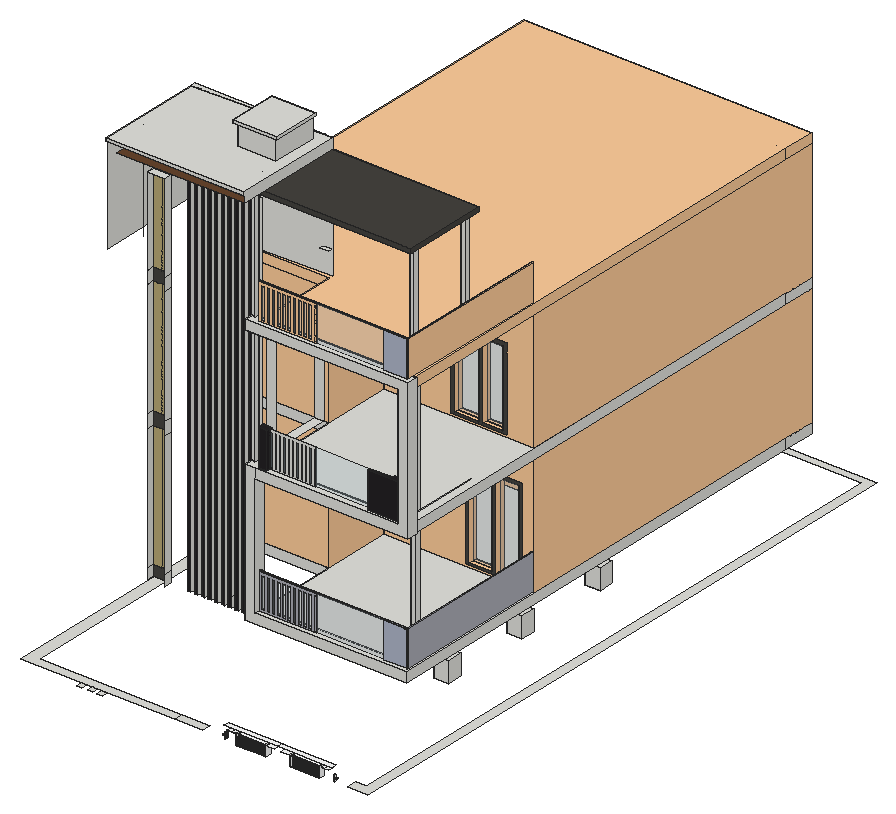
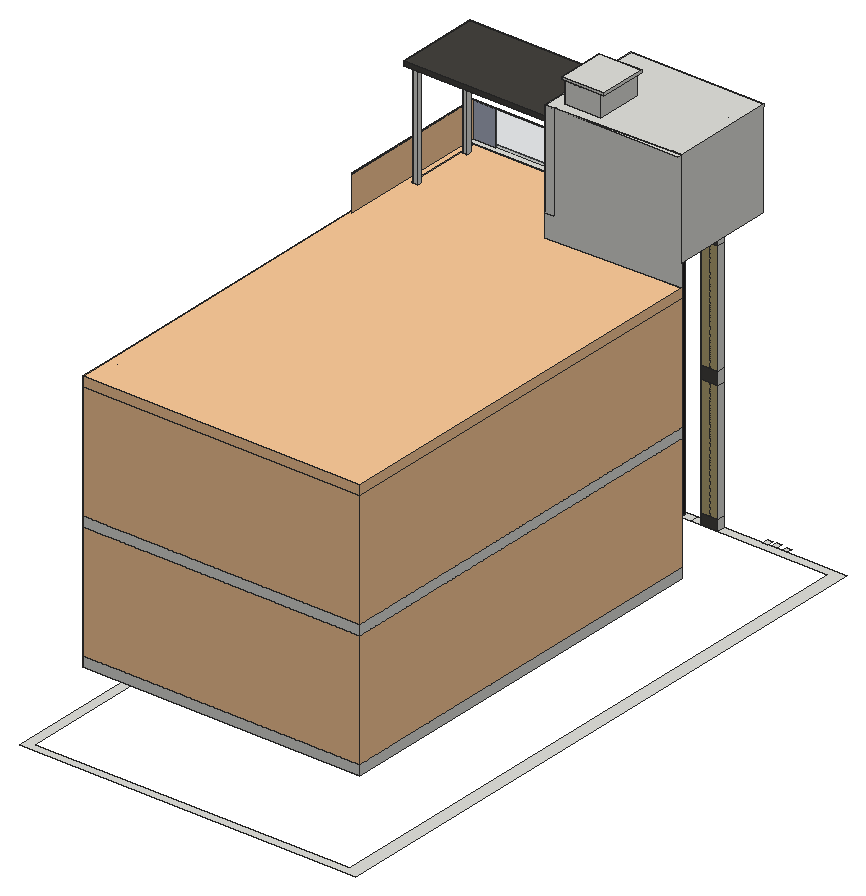
# SketchUp Ruby script. Lengths in inches.
U = 1.inch
M = Sketchup.active_model
def pt(a) = Geom::Point3d.new(a.map { |v| v * U })
def face(e, loops, mat)
  f = e.add_face(loops[0].map { |a| pt(a) })
  loops[1..].each { |l| e.add_face(l.map { |a| pt(a) }).erase! }
  f.material = f.back_material = mat if mat
  f
end
# faces: each face lists its corners as indices into pts; further lists are holes
def faces(e, pts, list, mat = nil) = list.each { |f| face(e, (f[0].is_a?(Array) ? f : [f]).map { |l| l.map { |i| pts[i] } }, mat) }
# xy, xz, yz: faces in a plane at the given z, y or x. An outline is a flat list of corners, or four numbers for a rectangle; further outlines are holes
def ring(l) = l.size == 4 ? [[l[0], l[1]], [l[2], l[1]], [l[2], l[3]], [l[0], l[3]]] : l.each_slice(2).to_a
def flat(e, list, mat, &to3) = list.each { |f| face(e, (f[0].is_a?(Array) ? f : [f]).map { |l| ring(l).map { |u, v| to3.(u, v) } }, mat) }
def xy(e, z, list, mat = nil) = flat(e, list, mat) { |x, y| [x, y, z] }
def xz(e, y, list, mat = nil) = flat(e, list, mat) { |x, z| [x, y, z] }
def yz(e, x, list, mat = nil) = flat(e, list, mat) { |y, z| [x, y, z] }
def lines(e, pts, list) = list.each { |a, b| e.add_line(pt(pts[a]), pt(pts[b])) }
# prism: a flat outline (further loops are holes) pulled along v
def prism(e, loops, v, mat = nil)
  f = face(e, loops, mat); d = Geom::Vector3d.new(v.map { |x| x * U })
  f.pushpull(f.normal.samedirection?(d) ? d.length : -d.length)
end
def box(e, o, s, mat = nil) = prism(e, [[o, [o[0] + s[0], o[1], o[2]], [o[0] + s[0], o[1] + s[1], o[2]], [o[0], o[1] + s[1], o[2]]]], [0, 0, s[2]], mat)
def at(x, y, z, deg = 0) = Geom::Transformation.translation(pt([x, y, z])) * Geom::Transformation.rotation(ORIGIN, Z_AXIS, deg.degrees)
def axes(o, x, y, z) = Geom::Transformation.new([*x, 0, *y, 0, *z, 0, *pt(o).to_a, 1])
def part(name) = M.definitions.add(name)
# library, detail: a bought-in or finely detailed component or shape, given as its bounding box
def library(name, o, s) = part(name).tap { |d| box(d.entities, o, s) }
def detail(e, o, s) = box(e.add_group.entities, o, s)
def put(e, d, t, mat = nil) = e.add_instance(d, t).tap { |i| i.material = mat if mat }
def group(e, t, mat = nil) = e.add_group.tap { |g| g.transformation = t; g.material = mat if mat }.entities
root = M.entities
M.materials.add("C02_Golden_Beige").color = [255, 205, 155]
M.materials.add("Glass_Basic_01").color = [161, 173, 186]
M.materials["Glass_Basic_01"].alpha = 0.25
M.materials.add("Glass_Mirror_01").color = [185, 168, 118]
M.materials.add("Glass_Safety_01").color = [204, 235, 244]
M.materials["Glass_Safety_01"].alpha = 0.25
M.materials.add("Marble_03_1K").color = [175, 182, 201]
M.materials.add("Marble_07_1K").color = [36, 34, 36]
M.materials.add("Marble_20_1K").color = [172, 173, 182]
M.materials.add("Wood_Planks_01_1K").color = [69, 67, 63]
M.materials.add("Wood_Veneer_15_1K").color = [103, 69, 45]
M.materials.add("[Color_000]").color = [255, 255, 255]
M.materials.add("[Color_C20]").color = [102, 91, 81]
c1 = part("Gate slat")
xy(c1.entities,0,[[0.39,114.16,6.3,114.17]])
xy(c1.entities,0,[[0.39,0,6.3,114.16]],"[Color_C20]")
xy(c1.entities,0.39,[[0.39,0,0.79,114.17],[0.98,0,2.07,114.17],[2.36,0,3.2,114.17],[3.59,0,4.37,114.17],[4.56,0,5.71,114.17],
  [5.91,0,6.3,114.17]],"[Color_C20]")
xy(c1.entities,0.79,[[0.39,0,0.79,114.17],[0.98,0,2.07,114.17],[2.36,0,3.2,114.17],[3.59,0,4.37,114.17],[4.56,0,5.71,114.17],
  [5.91,0,6.3,114.17]],"[Color_C20]")
xy(c1.entities,0.99,[[1.13,0,1.21,114.16],[1.87,0,1.94,114.16],[2.61,0,2.68,114.16],[3.35,0,3.42,114.16],[4.08,0,4.16,114.16],
  [4.82,0,4.9,114.16],[5.5625,0,5.63,114.16],[6.3,0,6.37,114.16]],"[Color_C20]")
xy(c1.entities,1.18,[[0.39,114.16,3.35,114.17],[3.35,114.16,6.3,114.17]])
xy(c1.entities,1.18,[[0.39,0,1.13,114.16],[1.21,0,1.87,114.16],[1.94,0,2.61,114.16],[2.68,0,3.35,114.16],[3.42,0,4.08,114.16],
  [4.16,0,4.82,114.16],[4.9,0,5.5625,114.16],[5.63,0,6.3,114.16]],"[Color_C20]")
xz(c1.entities,0,[[[0.39,0,6.3,0,6.3,0.39,5.91,0.39,5.91,0.79,6.3,0.79,6.3,1.18,5.63,1.18,5.63,0.99,5.5625,0.99,5.5625,1.18,4.9,1.18,4.9,0.99,4.82,0.99,4.82,1.18,4.16,1.18,4.16,0.99,4.08,0.99,4.08,1.18,3.42,1.18,3.42,0.99,3.35,0.99,3.35,1.18,2.68,1.18,2.68,0.99,2.61,0.99,2.61,1.18,1.94,1.18,1.94,0.99,1.87,0.99,1.87,1.18,1.21,1.18,1.21,0.99,1.13,0.99,1.13,1.18,0.39,1.18,0.39,0.79,0.79,0.79,0.79,0.39,0.39,0.39],[4.56,0.39,5.71,0.79],[0.98,0.39,2.07,0.79],[2.36,0.39,3.2,0.79],[3.59,0.39,4.37,0.79]],[6.3,0.99,6.37,1.18]],"[Color_C20]")
xz(c1.entities,114.16,[[1.13,0.99,1.21,1.18],[1.87,0.99,1.94,1.18],[2.61,0.99,2.68,1.18],[3.35,0.99,3.42,1.18],[4.08,0.99,4.16,1.18],
  [4.82,0.99,4.9,1.18],[5.5625,0.99,5.63,1.18]],"[Color_C20]")
xz(c1.entities,114.17,[[[0.39,0,0.39,0.39,0.79,0.39,0.79,0.79,0.39,0.79,0.39,1.18,6.3,1.18,6.3,0.79,5.91,0.79,5.91,0.39,6.3,0.39,6.3,0],[4.56,0.39,5.71,0.79],[0.98,0.39,2.07,0.79],[2.36,0.39,3.2,0.79],[3.59,0.39,4.37,0.79]]],"[Color_C20]")
yz(c1.entities,0.39,[[114.16,0,114.17,0.39],[114.16,0.79,114.17,1.18]])
yz(c1.entities,0.39,[[0,0,114.16,0.39],[0,0.79,114.16,1.18]],"[Color_C20]")
yz(c1.entities,0.79,[[0,0.39,114.17,0.79]],"[Color_C20]")
yz(c1.entities,0.98,[[0,0.39,114.17,0.79]],"[Color_C20]")
yz(c1.entities,1.13,[[0,0.99,114.16,1.18]],"[Color_C20]")
yz(c1.entities,1.21,[[0,0.99,114.16,1.18]],"[Color_C20]")
yz(c1.entities,1.87,[[0,0.99,114.16,1.18]],"[Color_C20]")
yz(c1.entities,1.94,[[0,0.99,114.16,1.18]],"[Color_C20]")
yz(c1.entities,2.07,[[0,0.39,114.17,0.79]],"[Color_C20]")
yz(c1.entities,2.36,[[0,0.39,114.17,0.79]],"[Color_C20]")
yz(c1.entities,2.61,[[0,0.99,114.16,1.18]],"[Color_C20]")
yz(c1.entities,2.68,[[0,0.99,114.16,1.18]],"[Color_C20]")
yz(c1.entities,3.2,[[0,0.39,114.17,0.79]],"[Color_C20]")
yz(c1.entities,3.35,[[0,0.99,114.16,1.18]],"[Color_C20]")
yz(c1.entities,3.42,[[0,0.99,114.16,1.18]],"[Color_C20]")
yz(c1.entities,3.59,[[0,0.39,114.17,0.79]],"[Color_C20]")
yz(c1.entities,4.08,[[0,0.99,114.16,1.18]],"[Color_C20]")
yz(c1.entities,4.16,[[0,0.99,114.16,1.18]],"[Color_C20]")
yz(c1.entities,4.37,[[0,0.39,114.17,0.79]],"[Color_C20]")
yz(c1.entities,4.56,[[0,0.39,114.17,0.79]],"[Color_C20]")
yz(c1.entities,4.82,[[0,0.99,114.16,1.18]],"[Color_C20]")
yz(c1.entities,4.9,[[0,0.99,114.16,1.18]],"[Color_C20]")
yz(c1.entities,5.5625,[[0,0.99,114.16,1.18]],"[Color_C20]")
yz(c1.entities,5.63,[[0,0.99,114.16,1.18]],"[Color_C20]")
yz(c1.entities,5.71,[[0,0.39,114.17,0.79]],"[Color_C20]")
yz(c1.entities,5.91,[[0,0.39,114.17,0.79]],"[Color_C20]")
yz(c1.entities,6.3,[[114.16,0,114.17,0.39],[114.16,0.79,114.17,1.18]])
yz(c1.entities,6.3,[[0,0,114.16,0.39],[0,0.79,114.16,0.99],[0,0.99,114.16,1.18]],"[Color_C20]")
yz(c1.entities,6.37,[[0,0.99,114.16,1.18]],"[Color_C20]")
p = [[0,0,0],[0.39,0,0]]
lines(c1.entities,p,[[0,1]])
c2 = part("Gate infill panel")
put(c2.entities,c1,axes([0,1.18,0],[3.67755,0,0],[0,0,2.40086],[0,-1,0]))
put(c2.entities,c1,axes([21.72,1.18,0],[3.67755,0,0],[0,0,2.40086],[0,-1,0]))
c3 = part("Balcony parapet")
xy(c3.entities,36.47,[[0,0,148.92,0,148.92,156.71,148.2,156.71,148.2,0.61,0,0.61]])
xz(c3.entities,0,[[148.53,0,148.92,0,148.92,36.47,0,36.47,0,36,148.53,36]])
xz(c3.entities,0.31,[[[0,0,57.9,0,57.9,1.37,55.24,1.37,55.24,32.37,57.9,32.37,57.9,36,0,36],[50.01,1.37,52.67,32.37],[44.78,1.37,47.44,32.37],[39.56,1.37,42.22,32.37],[34.33,1.37,36.99,32.37],[29.1,1.37,31.76,32.37],[23.87,1.37,26.53,32.37],[18.64,1.37,21.3,32.37],[13.42,1.37,16.08,32.37],[8.1875,1.37,10.85,32.37],[2.96,1.37,5.62,32.37]],[55.24,1.37,57.9,32.37]])
xz(c3.entities,0.31,[[57.9,0,124.92,36],[2.96,1.37,5.62,32.37],[8.1875,1.37,10.85,32.37],[13.42,1.37,16.08,32.37],[18.64,1.37,21.3,32.37],
  [23.87,1.37,26.53,32.37],[29.1,1.37,31.76,32.37],[34.33,1.37,36.99,32.37],[39.56,1.37,42.22,32.37],[44.78,1.37,47.44,32.37],
  [50.01,1.37,52.67,32.37]],"Glass_Basic_01")
xz(c3.entities,0.31,[[124.92,0,147.45,36]],"Marble_03_1K")
yz(c3.entities,148.73,[[0.31,0,156.71,36]])
yz(c3.entities,148.92,[[0,0,0.31,0,0.31,36,156.71,36,156.71,36.47,0,36.47]])
box(root,[422.82,488.53,99.54],[15.23,14.82,20.46])
box(root,[421,272.87,130],[4.67,4.67,127.6])
box(root,[421,272.87,258.55],[4.67,4.67,127.59])
box(root,[419.47,272.87,388.22],[4.67,4.67,110.73])
xy(root,57.7,[[324.17,176.2,351.84,181.72],[378.3125,176.2,405.98,181.35]],"[Color_000]")
xy(root,57.99,[[419.1,178.02,420.08,179.96],[310.07,178.15,311.05,180.23]],"[Color_000]")
xy(root,60.41,[[419.1,178.02,420.08,179.96],[310.07,178.15,311.05,180.23]],"[Color_000]")
xy(root,60.52,[[419.1,178.02,420.08,179.96],[420.08,178.02,422.11,179.96],[308.05,178.15,310.07,180.23],[310.07,178.15,311.05,180.23]],"[Color_000]")
xy(root,61.25,[[419.1,178.02,420.08,179.96],[420.08,178.02,422.11,179.96],[308.05,178.15,310.07,180.23],[310.07,178.15,311.05,180.23]],"[Color_000]")
xy(root,61.37,[[419.1,178.02,420.08,179.96],[310.07,178.15,311.05,180.23]],"[Color_000]")
xy(root,61.54,[[170.97,167.01,176.23,173.01],[181.8125,167.01,187.07,173.01],[191.24,167.01,196.49,173.01],[109.49,173.01,264.32,173.01,264.32,182.01,121.46,182.01,121.46,802.53,448.27,802.53,448.27,183.1,437.93,183.1,437.93,173.01,457.3,173.01,457.3,809.97,109.49,809.97],[264.32,173.01,291.9,182.01]])
xy(root,63.7,[[419.1,178.02,420.08,179.96],[310.07,178.15,311.05,180.23]],"[Color_000]")
xy(root,67.74,[[314.15,176.2,318.5,181.72],[318.5,176.2,322.85,181.72],[324.17,176.2,351.84,181.72],[353.16,176.2,361.87,181.72],[368.29,176.2,376.99,181.35],
  [378.3125,176.2,405.98,181.35],[407.3,176.2,411.65,181.35],[411.65,176.2,416,181.35]],"[Color_000]")
xy(root,71.31,[[311.05,176.2,364.96,181.72],[365.1875,176.2,419.1,181.35]],"[Color_000]")
xy(root,106.375,[[274.49,272.89,283.49,328.91]])
xy(root,120,[[209.38,257.97,212.62,260.97],[216.1875,257.97,219.55,260.97],[222.92,257.97,226.28,260.97],[229.65,257.97,233.01,260.97],[236.38,257.97,239.74,260.97],
  [243.11,257.97,246.47,260.97],[249.84,257.97,253.2,260.97],[256.57,257.97,259.93,260.97],[263.3,257.97,266.66,260.97],[270.03,257.97,273.39,260.97],
  [422.82,298.73,438.05,313.55],[422.82,390.01,438.05,404.84]])
xy(root,130,[[432.02,254.25,432.4,254.5625],[273.39,257.97,276.76,260.97],[280.12,257.97,283.49,260.97]])
xy(root,166,[[283.49,254.25,431.67,254.5625],[431.67,254.25,432.02,254.5625],[283.49,254.5625,431.67,254.87],[431.67,254.5625,431.67,254.87,431.6875,254.87,431.6875,255.07,432.02,255.07,432.02,254.5625],[432.02,254.5625,432.02,255.07,431.6875,255.07,431.6875,410.97,432.21,410.97,432.21,254.5625],
  [432.21,254.5625,432.4,410.97],[431.67,254.87,431.6875,255.07]])
xy(root,260,[[285.04,252.1,293.12,258.44],[394.1875,252.1,394.1875,255.27,416.46,255.27,416.46,258.44,424.55,258.44,424.55,252.1]])
xy(root,264.75,[[274.49,275.82,283.49,335.125]])
xy(root,296,[[285.04,252.1,293.12,258.44],[394.1875,252.1,424.55,252.1,424.55,258.44,416.46,258.44,416.46,255.27,394.1875,255.27]],"Marble_07_1K")
xy(root,370.51,[[274.49,275.82,283.49,335.125]])
xy(root,388.22,[[419.47,337.16,424.14,341.83]])
xy(root,414,[[274.49,341.97,283.49,346.68]])
xy(root,485.41,[[172.32,253.51,190.09,260.97]])
xy(root,498.95,[[209.38,257.97,212.62,260.97],[216.1875,257.97,219.55,260.97],[222.92,257.97,226.28,260.97],[229.65,257.97,233.01,260.97],[236.38,257.97,239.74,260.97],
  [243.11,257.97,246.47,260.97],[249.84,257.97,253.2,260.97],[256.57,257.97,259.93,260.97],[263.3,257.97,266.66,260.97],[270.03,257.97,273.39,260.97],
  [273.39,257.97,276.76,260.97],[280.12,257.97,283.49,260.97],[419.47,337.16,424.14,341.83]])
xy(root,498.95,[[[283.49,260.97,429.93,346.68],[419.47,337.16,424.14,341.83]]],"Wood_Planks_01_1K")
xy(root,503.43,[[283.49,260.97,429.93,346.68]],"Wood_Planks_01_1K")
xy(root,503.43,[[154.49,236.97,154.49,253.51,209.38,253.51,209.38,260.97,283.49,260.97,283.49,236.97]],"Wood_Veneer_15_1K")
xy(root,511.11,[[145.49,234.97,283.49,236.97]])
xy(root,514.11,[[[145.49,234.97,283.49,234.97,283.49,346.68,274.49,346.38,145.49,341.97],[234.33,289.4,272.3,335.31]],[145.49,341.97,274.49,346.38,274.49,346.68,145.49,346.68],[274.49,346.38,283.49,346.68,274.49,346.68]])
xy(root,535.5625,[[231.33,286.4,275.3,289.4],[231.33,289.4,234.33,335.31],[234.33,289.4,272.3,335.31],[272.3,289.4,275.3,335.31]])
xy(root,538.11,[[231.33,286.4,275.3,335.31]])
xz(root,176.2,[[322.85,57.7,324.17,67.74],[351.84,57.7,353.16,67.74],[376.99,57.7,378.3125,67.74],[405.98,57.7,407.3,67.74]],"[Color_000]")
xz(root,178.02,[[419.1,57.99,420.08,60.41],[419.1,60.52,422.11,61.25],[419.1,61.37,420.08,63.7]],"[Color_000]")
xz(root,178.15,[[310.07,57.99,311.05,60.41],[308.05,60.52,311.05,61.25],[310.07,61.37,311.05,63.7]],"[Color_000]")
xz(root,179.96,[[419.1,57.99,420.08,60.41],[419.1,60.52,420.08,60.81],[420.08,60.52,420.08,60.81,419.1,60.81,419.1,61.25,422.11,61.25,422.11,60.52],[419.1,61.37,420.08,63.7]],"[Color_000]")
xz(root,180.23,[[310.07,57.99,311.05,60.41],[308.05,60.52,308.05,61.25,311.05,61.25,311.05,60.81,310.07,60.81,310.07,60.52],[310.07,60.52,311.05,60.81],[310.07,61.37,311.05,63.7]],"[Color_000]")
xz(root,234.97,[[145.49,511.11,283.49,514.11]])
xz(root,252.1,[[285.04,260,293.12,296],[394.1875,260,424.55,296]],"Marble_07_1K")
xz(root,254.5625,[[432.02,130,432.21,166],[432.21,130,432.4,166]])
xz(root,254.87,[[283.49,166,431.6875,166.47]])
xz(root,255.27,[[[293.12,260,339.78,260,339.78,261.51,338.37,261.51,338.37,293.3,339.78,293.3,339.78,296,293.12,296],[334.01,261.51,335.43,293.3],[329.66,261.51,331.07,293.3],[325.3,261.51,326.72,293.3],[320.94,261.51,322.36,293.3],[316.59,261.51,318.01,293.3],[312.23,261.51,313.65,293.3],[307.88,261.51,309.3,293.3],[303.52,261.51,304.94,293.3],[299.17,261.51,300.59,293.3],[294.8125,261.51,296.23,293.3]],[338.37,261.51,339.78,293.3]])
xz(root,255.27,[[339.78,260,394.1875,296],[294.8125,261.51,296.23,293.3],[299.17,261.51,300.59,293.3],[303.52,261.51,304.94,293.3],[307.88,261.51,309.3,293.3],
  [312.23,261.51,313.65,293.3],[316.59,261.51,318.01,293.3],[320.94,261.51,322.36,293.3],[325.3,261.51,326.72,293.3],[329.66,261.51,331.07,293.3],
  [334.01,261.51,335.43,293.3]],"Glass_Safety_01")
xz(root,255.27,[[394.1875,260,416.46,296]],"Marble_07_1K")
xz(root,257.97,[[273.39,130,276.76,498.95],[280.12,130,283.49,498.95]])
xz(root,257.97,[[209.38,120,212.62,498.95],[216.1875,120,219.55,498.95],[222.92,120,226.28,498.95],[229.65,120,233.01,498.95],[236.38,120,239.74,498.95],
  [243.11,120,246.47,498.95],[249.84,120,253.2,498.95],[256.57,120,259.93,498.95],[263.3,120,266.66,498.95],[270.03,120,273.39,498.95]],"Marble_07_1K")
xz(root,258.44,[[285.04,260,293.12,296],[416.46,260,424.55,296]],"Marble_07_1K")
xz(root,260.97,[[172.32,130,181.21,254.15],[181.21,130,190.09,254.15],[172.32,267.51,181.21,383.98],[181.21,267.51,190.09,383.98],[172.32,396.42,181.21,485.41],
  [181.21,396.42,190.09,485.41]],"Glass_Mirror_01")
xz(root,260.97,[[276.76,130,280.12,498.95]],"Marble_07_1K")
xz(root,260.97,[[172.32,119.26,190.09,130],[172.32,254.15,190.09,267.51],[172.32,383.98,190.09,396.42],[209.38,498.95,429.93,503.43]],"Wood_Planks_01_1K")
xz(root,275.82,[[274.49,264.75,283.49,370.51]])
xz(root,286.4,[[231.33,535.5625,275.3,538.11]])
xz(root,289.4,[[234.33,514.11,272.3,535.5625]])
xz(root,298.73,[[422.82,99.54,438.05,120]])
xz(root,335.125,[[274.49,264.75,283.49,370.51]])
xz(root,335.31,[[234.33,514.11,272.3,535.5625],[231.33,535.5625,275.3,538.11]])
xz(root,337.16,[[419.47,388.22,424.14,498.95]])
xz(root,341.83,[[419.47,388.22,424.14,498.95]])
xz(root,341.97,[[145.49,414,154.73,514.11]])
xz(root,346.68,[[274.49,414,283.49,514.11]])
xz(root,346.68,[[283.49,498.95,429.93,503.43]],"Wood_Planks_01_1K")
xz(root,390.01,[[422.82,99.54,438.05,120]])
xz(root,410.97,[[431.6875,166,432.4,166.47]])
yz(root,145.49,[[236.97,414,236.97,511.11,234.97,511.11,234.97,514.11,341.97,514.11,341.97,414]])
yz(root,172.32,[[253.51,119.26,260.97,130],[253.51,130,260.97,254.15],[253.51,254.15,260.97,267.51],[253.51,267.51,260.97,383.98],[253.51,383.98,260.97,396.42],
  [253.51,396.42,260.97,485.41]])
yz(root,190.09,[[253.51,119.26,260.97,130],[253.51,130,260.97,254.15],[253.51,254.15,260.97,267.51],[253.51,267.51,260.97,383.98],[253.51,383.98,260.97,396.42],
  [253.51,396.42,260.97,485.41]])
yz(root,212.62,[[257.97,120,260.97,498.95]])
yz(root,216.1875,[[257.97,120,260.97,498.95]])
yz(root,219.55,[[257.97,120,260.97,498.95]])
yz(root,222.92,[[257.97,120,260.97,498.95]])
yz(root,226.28,[[257.97,120,260.97,498.95]])
yz(root,229.65,[[257.97,120,260.97,498.95]])
yz(root,231.33,[[286.4,535.5625,335.31,538.11]])
yz(root,233.01,[[257.97,120,260.97,498.95]])
yz(root,234.33,[[289.4,514.11,335.31,535.5625]])
yz(root,236.38,[[257.97,120,260.97,498.95]])
yz(root,239.74,[[257.97,120,260.97,498.95]])
yz(root,243.11,[[257.97,120,260.97,498.95]])
yz(root,246.47,[[257.97,120,260.97,498.95]])
yz(root,249.84,[[257.97,120,260.97,498.95]])
yz(root,253.2,[[257.97,120,260.97,130],[257.97,130,260.97,498.95]])
yz(root,256.57,[[257.97,120,260.97,498.95]])
yz(root,259.93,[[257.97,120,260.97,498.95]])
yz(root,263.3,[[257.97,120,260.97,498.95]])
yz(root,266.66,[[257.97,120,260.97,498.95]])
yz(root,270.03,[[257.97,120,260.97,498.95]])
yz(root,272.3,[[289.4,514.11,335.31,535.5625]])
yz(root,273.39,[[257.97,120,260.97,130]])
yz(root,275.3,[[286.4,535.5625,335.31,538.11]])
yz(root,276.76,[[257.97,130,260.97,498.95]])
yz(root,280.12,[[257.97,130,260.97,498.95]])
yz(root,283.49,[[254.25,166,254.87,166.47],[236.97,503.43,346.68,503.43,346.68,514.11,234.97,514.11,234.97,511.11,236.97,511.11]])
yz(root,285.04,[[252.1,260,258.44,296]],"Marble_07_1K")
yz(root,293.12,[[252.1,260,255.27,296],[255.27,260,258.44,296]],"Marble_07_1K")
yz(root,308.05,[[178.15,60.52,180.23,61.25]],"[Color_000]")
yz(root,310.07,[[178.15,57.99,180.23,60.41],[178.15,61.37,180.23,63.7]],"[Color_000]")
yz(root,322.85,[[176.2,57.7,181.72,67.74]],"[Color_000]")
yz(root,324.17,[[176.2,57.7,181.72,67.74]],"[Color_000]")
yz(root,351.84,[[176.2,57.7,181.72,67.74]],"[Color_000]")
yz(root,353.16,[[176.2,57.7,181.72,67.74]],"[Color_000]")
yz(root,376.99,[[176.2,57.7,181.35,67.74]],"[Color_000]")
yz(root,378.3125,[[176.2,57.7,181.35,67.74]],"[Color_000]")
yz(root,394.1875,[[252.1,260,255.27,296]],"Marble_07_1K")
yz(root,405.98,[[176.2,57.7,181.35,67.74]],"[Color_000]")
yz(root,407.3,[[176.2,57.7,181.35,67.74]],"[Color_000]")
yz(root,416.46,[[255.27,260,258.44,296]],"Marble_07_1K")
yz(root,419.47,[[337.16,388.22,341.83,498.95]])
yz(root,420.08,[[178.02,57.99,179.96,60.41],[178.02,61.37,179.96,63.7]],"[Color_000]")
yz(root,422.82,[[298.73,99.54,313.55,120],[390.01,99.54,404.84,120]])
yz(root,424.14,[[337.16,388.22,341.83,498.95]])
yz(root,424.55,[[252.1,260,258.44,296]])
yz(root,429.93,[[260.97,498.95,346.68,503.43]],"Wood_Planks_01_1K")
yz(root,431.6875,[[254.87,166,410.97,166.47]])
yz(root,432.02,[[254.25,130,254.5625,166]])
yz(root,438.05,[[298.73,99.54,313.55,120],[390.01,99.54,404.84,120]])
p = [[274.49,346.38,514.11],[283.49,346.68,514.11],[283.49,346.68,503.43],[283.49,346.68,498.95],[283.49,346.68,414],[283.49,346.68,390],
  [145.49,341.97,390],[145.49,341.97,414],[145.49,341.97,514.11],[154.73,269.97,414],[154.73,269.97,514.11],[274.49,269.97,414],
  [274.49,269.97,514.11],[410.03,177.06,67.73],[378.3125,177.06,67.73],[320.12,177.12,67.73],[351.84,177.12,67.73],[311.05,180.23,60.52],
  [311.05,180.23,60.41]]
faces(root,p,[[0,1,2,3,4,5,6,7,8]])
lines(root,p,[[9,10],[11,12],[13,14],[15,16],[17,18]])
put(root,c2,axes([378.3125,177.06,57.09],[0,0,0.23699],[0,0.34901,0],[0.10093,0,0]))
put(root,c2,axes([351.84,177.12,57.09],[0,0,0.23699],[0,0.374,0],[-0.10093,0,0]))
g1 = group(root,at(145.49,341.97,120))
xy(g1,0,[[127.934,-92.359,127.897,-81.525,280.269,-81,280.321,-81,280.599,-80.999,280.598,-80.828,280.32,0,280.042,-0.001,280.32,-80.56,280.321,-80.829,280.32,-81,138,-81,138,0,0,0,0,417,288,417,288,383.393,279,383.362,288,383.362,289.636,-91.802],[280.321,-81,280.321,-80.829,280.598,-80.828,280.599,-80.999],[280.321,-80.829,280.32,-80.56,280.32,0,280.598,-80.828],[280.32,-80.56,280.042,-0.001,280.32,0],[279,383.362,288,383.393,288,383.364,287.403,383.362],
  [287.403,383.362,288,383.364,288,383.362]])
xy(g1,10,[[138,-92.324,289.636,-91.802,288,383.362,287.403,383.362,288,383.364,288,417,0,417,0,0,138,0,138,-81,280.32,-81,280.321,-80.829,280.321,-81,280.269,-81,127.905,-81.525,127.897,-81.525,127.905,-84,127.905,-81.525,138,-81.525],[287.403,383.362,288,383.362,288,383.364]])
xy(g1,130.168,[[138,-92.324,291.281,-81.525]])
xy(g1,140,[[127.934,-92.359,138,-92.324,280.825,-92.324,280.825,-81.525,127.905,-81.525,127.905,-84]])
xy(g1,260.817,[[127.934,-92.324,280.825,-81.525]])
xy(g1,270,[[127.934,-92.324,291.281,-81.525]])
xz(g1,-92.324,[[138,130.168,291.281,130.168,291.281,270,127.934,270,127.934,260.817,280.825,260.817,280.825,140,138,140]])
xz(g1,-81.525,[[127.905,10,127.905,140,280.825,140,280.825,260.817,127.934,260.817,127.934,270,291.281,270,291.281,130.168,138,130.168,138,10]])
xz(g1,-81,[[138,0,280.269,10],[280.269,0,280.32,10],[280.32,0,280.321,10]])
xz(g1,0,[[0,0,138,10]])
xz(g1,417,[[0,0,288,10]])
yz(g1,0,[[0,0,417,10]])
yz(g1,127.905,[[-84,10,-81.525,140]])
yz(g1,127.934,[[-92.324,260.817,-81.525,270]])
yz(g1,138,[[-81,0,0,10],[-92.324,10,-81.525,130.168]])
yz(g1,280.321,[[-81,0,-80.829,10]])
yz(g1,280.825,[[-92.324,140,-81.525,260.817]])
yz(g1,288,[[383.362,0,383.393,10],[383.393,0,417,10]])
yz(g1,291.281,[[-92.324,130.168,-81.525,270]])
p = [[289.636,-91.802,10],[138,-92.324,10],[138,-92.324,130.168],[138,-92.324,140],[127.934,-92.359,140],[127.934,-92.359,0],
  [289.636,-91.802,0],[127.905,-84,10],[127.897,-81.525,10],[127.897,-81.525,0],[127.905,-84,140],[288,383.362,0],
  [288,383.362,10],[280.269,-81,10],[280.269,-81,0],[127.905,-81.525,10],[280.32,-81,0],[280.321,-80.829,0],
  [280.321,-80.829,10],[280.32,-81,10],[280.32,0,10],[280.32,0,0],[280.042,-0.001,0],[280.042,-0.001,10],
  [279,383.362,10],[279,383.362,0],[280.598,-80.828,10],[280.598,-80.828,0]]
faces(g1,p,[[0,1,2,3,4,5,6],[7,8,9,5,4,10],[6,11,12,0],[13,14,9,8,15],[16,17,18,19],[20,21,22,23]])
lines(g1,p,[[24,25],[26,27]])
put(root,c3,at(283.49,254.25,130),"Marble_20_1K")
g2 = group(root,at(145.49,341.97,130),"C02_Golden_Beige")
xy(g2,0,[[9,9,129,9,129,198,279,198,279,408,9,408],[138,69,138,78,279,78,279,189,288,189,288,69]])
xy(g2,3.63,[[223.16,69,246.125,73.5],[246.125,69,250.37,78],[250.37,69,272.65,73.5],[223.16,73.5,246.125,78],[250.37,73.5,272.65,78]])
xy(g2,91.02,[[223.16,69,246.125,73.5],[250.37,69,272.65,73.5],[223.16,73.5,246.125,78],[250.37,73.5,272.65,78]])
xy(g2,120,[[[0,0,138,0,138,69,288,69,288,417,0,417],[9,9,9,408,279,408,279,78,138,78,138,189,279,189,279,198,129,198,129,9]]])
xz(g2,0,[[0,0,138,120]])
xz(g2,9,[[9,0,129,120]])
xz(g2,69,[[[138,0,288,120],[218.42,1.1,277.11,95.02]]])
xz(g2,69,[[[218.42,1.1,277.11,95.02],[223.16,3.63,246.125,91.02],[250.37,3.63,272.65,91.02]]],"Wood_Planks_01_1K")
xz(g2,73.5,[[223.16,3.63,246.125,91.02],[250.37,3.63,272.65,91.02]],"Glass_Basic_01")
xz(g2,78,[[[138,0,279,120],[223.16,3.63,246.125,91.02],[250.37,3.63,272.65,91.02]]])
xz(g2,189,[[138,0,279,120]])
xz(g2,198,[[129,0,138,120],[138,0,279,120]])
xz(g2,408,[[9,0,279,120]])
xz(g2,417,[[0,0,288,120]])
yz(g2,0,[[0,0,417,120]])
yz(g2,9,[[9,0,408,120]])
yz(g2,129,[[9,0,198,120]])
yz(g2,138,[[0,0,69,120],[69,0,78,120],[78,0,189,120]])
yz(g2,223.16,[[69,3.63,73.5,91.02],[73.5,3.63,78,91.02]])
yz(g2,246.125,[[69,3.63,73.5,91.02],[73.5,3.63,78,91.02]])
yz(g2,250.37,[[69,3.63,73.5,91.02],[73.5,3.63,78,91.02]])
yz(g2,272.65,[[69,3.63,73.5,91.02],[73.5,3.63,78,91.02]])
yz(g2,279,[[78,0,189,120],[189,0,198,120],[198,0,408,120]])
yz(g2,288,[[69,0,417,120]])
p = [[223.16,69,91.02],[218.42,69,91.02]]
lines(g2,p,[[0,1]])
g3 = group(root,at(145.49,341.97,250))
xy(g3,0,[[138,-81,138,0,0,0,0,417,288,417,288,383.393,279,383.362,288,383.362,289.598,-80.875,280.598,-80.906,280.32,0,280.32,-81],[279,383.362,288,383.393,288,383.364,287.403,383.362],[287.403,383.362,288,383.364,288,383.362]])
xy(g3,10,[[138,-81,280.32,-81,280.32,0,280.598,-80.906,289.598,-80.875,288,383.362,287.403,383.362,288,383.364,288,417,0,417,0,0,138,0],[287.403,383.362,288,383.362,288,383.364]])
xz(g3,-81,[[138,0,280.32,10]])
xz(g3,0,[[0,0,138,10]])
xz(g3,417,[[0,0,288,10]])
yz(g3,0,[[0,0,417,10]])
yz(g3,138,[[-81,0,0,10]])
yz(g3,280.32,[[-81,0,0,10]])
yz(g3,288,[[383.362,0,383.393,10],[383.393,0,417,10]])
p = [[280.32,0,10],[280.32,0,0],[280.598,-80.906,0],[280.598,-80.906,10],[289.598,-80.875,10],[289.598,-80.875,0],
  [288,383.362,0],[288,383.362,10],[279,383.362,10],[279,383.362,0]]
faces(g3,p,[[0,1,2,3],[4,3,2,5],[5,6,7,4]])
lines(g3,p,[[8,9]])
g4 = group(root,at(145.49,341.97,260),"C02_Golden_Beige")
xy(g4,0,[[9,9,129,9,129,198,279,198,279,408,9,408],[138,69,138,78,279,78,279,189,288,189,288,69]])
xy(g4,4.2,[[208.73,69,233.07,73.5],[237.18,69,257.4,73.5],[208.73,73.5,233.07,78],[237.18,73.5,257.4,78]])
xy(g4,80.99,[[208.73,69,233.07,73.5],[233.07,69,237.18,78],[237.18,69,257.4,73.5],[208.73,73.5,233.07,78],[237.18,73.5,257.4,78]])
xy(g4,120,[[[0,0,138,0,138,69,288,69,288,417,0,417],[9,9,9,408,279,408,279,78,138,78,138,189,279,189,279,198,129,198,129,9]]])
xz(g4,0,[[0,0,138,120]])
xz(g4,9,[[9,0,129,120]])
xz(g4,69,[[[138,0,288,120],[204.97,1.96,260.64,84.92]]])
xz(g4,69,[[[204.97,1.96,260.64,84.92],[208.73,4.2,233.07,80.99],[237.18,4.2,257.4,80.99]]],"Wood_Planks_01_1K")
xz(g4,73.5,[[208.73,4.2,233.07,80.99],[237.18,4.2,257.4,80.99]],"Glass_Basic_01")
xz(g4,78,[[[138,0,279,120],[208.73,4.2,233.07,80.99],[237.18,4.2,257.4,80.99]]])
xz(g4,189,[[138,0,279,120]])
xz(g4,198,[[129,0,138,120],[138,0,279,120]])
xz(g4,408,[[9,0,279,120]])
xz(g4,417,[[0,0,288,120]])
yz(g4,0,[[0,0,417,120]])
yz(g4,9,[[9,0,408,120]])
yz(g4,129,[[9,0,198,120]])
yz(g4,138,[[0,0,69,120],[69,0,78,120],[78,0,189,120]])
yz(g4,208.73,[[69,4.2,73.5,80.99],[73.5,4.2,78,80.99]])
yz(g4,233.07,[[69,4.2,73.5,80.99],[73.5,4.2,78,80.99]])
yz(g4,237.18,[[69,4.2,73.5,80.99],[73.5,4.2,78,80.99]])
yz(g4,257.4,[[69,4.2,73.5,80.99],[73.5,4.2,78,80.99]])
yz(g4,279,[[78,0,189,120],[189,0,198,120],[198,0,408,120]])
yz(g4,288,[[69,0,417,120]])
g5 = group(root,at(145.49,341.97,380),"C02_Golden_Beige")
xy(g5,0,[[138,-81,138,0,0,0,0,417,288,417,288,383.393,279,383.362,288,383.362,289.598,-80.968,280.599,-80.999,280.32,0,280.32,-81],[279,383.362,288,383.393,288,383.364,287.403,383.362],[287.403,383.362,288,383.364,288,383.362]])
xy(g5,10,[[138,-81,280.32,-81,280.32,0,280.599,-80.999,289.598,-80.968,288,383.362,287.403,383.362,288,383.364,288,417,0,417,0,0,138,0],[287.403,383.362,288,383.362,288,383.364]])
xz(g5,-81,[[138,0,280.32,10]])
xz(g5,0,[[0,0,138,10]])
xz(g5,417,[[0,0,288,10]])
yz(g5,0,[[0,0,417,10]])
yz(g5,138,[[-81,0,0,10]])
yz(g5,280.32,[[-81,0,0,10]])
yz(g5,288,[[383.362,0,383.393,10],[383.393,0,417,10]])
p = [[280.32,0,10],[280.32,0,0],[280.599,-80.999,0],[280.599,-80.999,10],[289.598,-80.968,0],[289.598,-80.968,10],
  [288,383.362,0],[288,383.362,10],[279,383.362,10],[279,383.362,0]]
faces(g5,p,[[0,1,2,3],[3,2,4,5],[4,6,7,5]])
lines(g5,p,[[8,9]])
put(root,c3,at(283.49,254.25,390),"C02_Golden_Beige")
